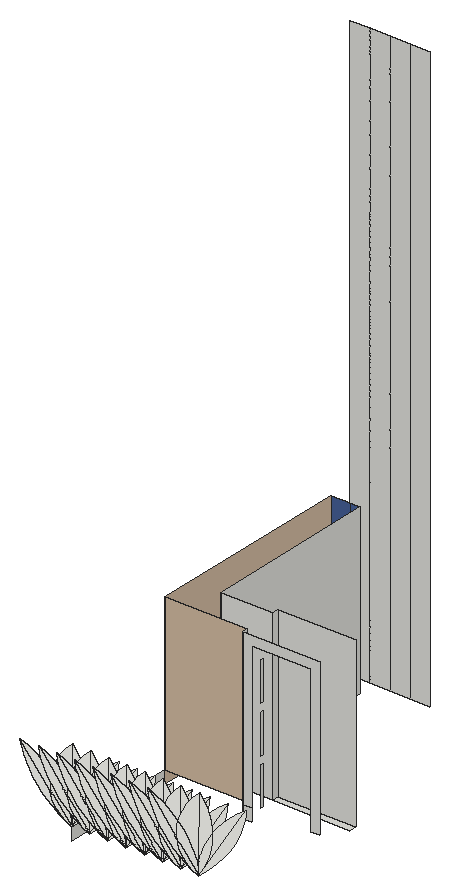
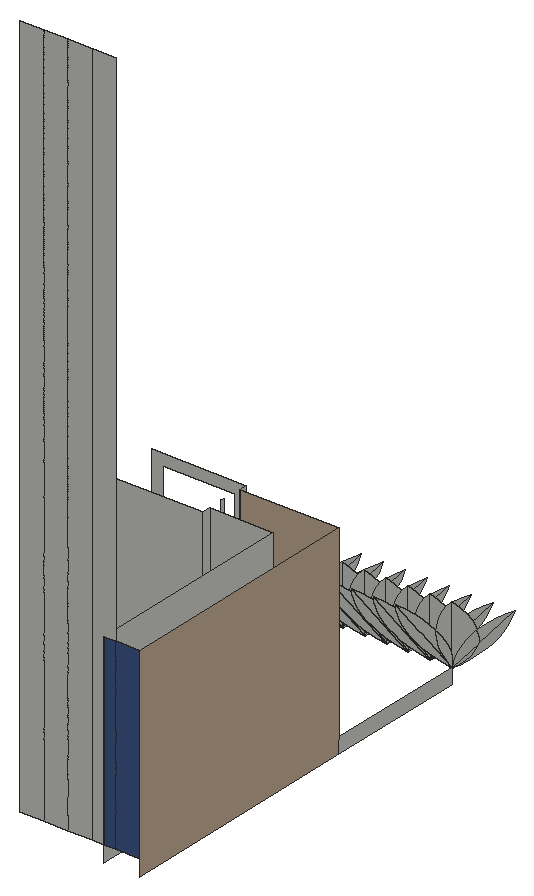
# SketchUp Ruby script. Lengths in inches.
U = 1.inch
M = Sketchup.active_model
def pt(a) = Geom::Point3d.new(a.map { |v| v * U })
def face(e, loops, mat)
  f = e.add_face(loops[0].map { |a| pt(a) })
  loops[1..].each { |l| e.add_face(l.map { |a| pt(a) }).erase! }
  f.material = f.back_material = mat if mat
  f
end
# faces: each face lists its corners as indices into pts; further lists are holes
def faces(e, pts, list, mat = nil) = list.each { |f| face(e, (f[0].is_a?(Array) ? f : [f]).map { |l| l.map { |i| pts[i] } }, mat) }
# xy, xz, yz: faces in a plane at the given z, y or x. An outline is a flat list of corners, or four numbers for a rectangle; further outlines are holes
def ring(l) = l.size == 4 ? [[l[0], l[1]], [l[2], l[1]], [l[2], l[3]], [l[0], l[3]]] : l.each_slice(2).to_a
def flat(e, list, mat, &to3) = list.each { |f| face(e, (f[0].is_a?(Array) ? f : [f]).map { |l| ring(l).map { |u, v| to3.(u, v) } }, mat) }
def xy(e, z, list, mat = nil) = flat(e, list, mat) { |x, y| [x, y, z] }
def xz(e, y, list, mat = nil) = flat(e, list, mat) { |x, z| [x, y, z] }
def yz(e, x, list, mat = nil) = flat(e, list, mat) { |y, z| [x, y, z] }
def lines(e, pts, list) = list.each { |a, b| e.add_line(pt(pts[a]), pt(pts[b])) }
# prism: a flat outline (further loops are holes) pulled along v
def prism(e, loops, v, mat = nil)
  f = face(e, loops, mat); d = Geom::Vector3d.new(v.map { |x| x * U })
  f.pushpull(f.normal.samedirection?(d) ? d.length : -d.length)
end
def box(e, o, s, mat = nil) = prism(e, [[o, [o[0] + s[0], o[1], o[2]], [o[0] + s[0], o[1] + s[1], o[2]], [o[0], o[1] + s[1], o[2]]]], [0, 0, s[2]], mat)
def at(x, y, z, deg = 0) = Geom::Transformation.translation(pt([x, y, z])) * Geom::Transformation.rotation(ORIGIN, Z_AXIS, deg.degrees)
def axes(o, x, y, z) = Geom::Transformation.new([*x, 0, *y, 0, *z, 0, *pt(o).to_a, 1])
def part(name) = M.definitions.add(name)
# library, detail: a bought-in or finely detailed component or shape, given as its bounding box
def library(name, o, s) = part(name).tap { |d| box(d.entities, o, s) }
def detail(e, o, s) = box(e.add_group.entities, o, s)
def put(e, d, t, mat = nil) = e.add_instance(d, t).tap { |i| i.material = mat if mat }
def group(e, t, mat = nil) = e.add_group.tap { |g| g.transformation = t; g.material = mat if mat }.entities
root = M.entities
M.materials.add("[Formica Blue]").color = [71, 97, 152]
M.materials.add("[Formica Laminate Light]").color = [213, 189, 164]
xy(root,-6,[[60.83,69.27,96.11,72.34]])
xz(root,52.17,[[60.83,-6,65.07,-0.3125],[60.83,-0.3125,65.07,-0.3125,65.07,66.01,91.875,66.01,91.875,-0.3125,96.11,-0.3125,96.11,70.25,60.83,70.25]])
xz(root,54.73,[[23.53,-0.3125,60.83,70.25]],"[Formica Laminate Light]")
xz(root,69.27,[[36.96,-6,60.83,70.25]])
xz(root,72.34,[[60.83,-6,96.11,70.25]])
xz(root,148.73,[[36.96,0,41.3,0,41.3,267.125,32.53,267.125,32.53,70.25,36.96,70.25],[41.3,0,50.53,267.125],[50.53,0,59.53,267.125],[59.53,0,68.53,267.125]])
xz(root,148.73,[[23.53,0,32.53,70.25],[32.53,0,36.96,70.25]],"[Formica Blue]")
yz(root,23.53,[[1.54,-6,54.73,-0.3125]])
yz(root,23.53,[[54.73,-6,148.73,70.25]],"[Formica Laminate Light]")
yz(root,36.96,[[69.27,-6,148.73,70.25]])
yz(root,60.83,[[52.17,-6,54.73,-0.3125],[69.27,-6,72.34,70.25],[52.17,-0.3125,54.73,70.25]])
yz(root,70.01,[[51.17,2,52.17,19.625],[51.17,23.34,52.17,40.97],[51.17,44.6875,52.17,62.3125]])
p = [[58.1,2.21,24.34],[56.99,2.71,26.88],[70.57,2.65,10.87],[70.7,2.54,10.46],[71.91,2.12,7.97],[73.51,1.91,5.5625],
  [75.51,1.92,3.27],[77.85,2.15,1.11],[80.53,2.6,-0.87],[77.79,2.13,1.125],[75.17,1.74,3.19],[72.6875,1.4375,5.33],
  [70.34,1.22,7.53],[68.13,1.1,9.79],[66.07,1.0625,12.1],[64.16,1.12,14.47],[62.41,1.26,16.88],[60.81,1.49,19.33],
  [59.37,1.81,21.82],[74.2,10.8125,27.37],[79.4,4.0625,4.15],[79.43,3.87,3.62],[79.84,3.17,1.37],[79.62,3.2,1.71],
  [78.5,3.7,4.27],[77.18,4.08,6.8],[75.66,4.36,9.28],[73.95,4.54,11.72],[72.04,4.6,14.11],[69.96,4.55,16.43],
  [69.6,4.53,16.79],[69.64,5.06,18.08],[70.15,6.27,20.56],[71.09,7.64,22.96],[72.45,9.17,25.23],[69.56,4.02,15.55],
  [69.92,3.18,12.99],[79.3125,4.69,5.86],[79.48,5.65,8.08],[79.9375,6.72,10.27],[80.68,7.9,12.4],[81.48,8.9,14.02],
  [81.65,8.74,13.4],[82.07,7.98,10.98],[82.25,7.11,8.56],[82.18,6.13,6.15],[81.87,5.05,3.77],[81.32,3.87,1.43],
  [88.37,15.11,21.72],[90.63,16.73,23.22],[81.7,9.18,14.46],[82.99,10.55,16.44],[84.54,12,18.32],[86.34,13.52,20.08],
  [90.9375,16.01,21.01],[91.03,15.18,18.81],[90.91,14.27,16.62],[90.57,13.26,14.46],[90.02,12.17,12.33],[89.26,11,10.25],
  [88.3,9.76,8.22],[87.13,8.44,6.25],[85.76,7.0625,4.34],[84.2,5.625,2.52],[82.45,4.14,0.78],[49.96,2.0625,24.42],
  [48.85,2.55,26.96],[62.43,2.5,10.95],[62.56,2.39,10.54],[63.76,1.97,8.05],[65.37,1.76,5.64],[67.36,1.77,3.35],
  [69.71,2,1.19],[72.39,2.45,-0.79],[69.64,1.98,1.21],[67.03,1.59,3.27],[64.54,1.29,5.41],[62.2,1.07,7.61],
  [59.99,0.95,9.87],[57.93,0.91,12.18],[56.02,0.96,14.55],[54.26,1.11,16.96],[52.67,1.34,19.41],[51.23,1.66,21.9],
  [61.42,3.87,15.625],[61.46,4.38,16.87],[61.8125,4.4,16.51],[63.9,4.45,14.1875],[65.81,4.38,11.8],[67.52,4.21,9.36],
  [69.04,3.93,6.875],[70.36,3.54,4.35],[71.48,3.05,1.79],[61.77,3.03,13.07],[66.06,10.66,27.45],[71.26,3.91,4.23],
  [71.29,3.71,3.7],[71.69,3.02,1.45],[61.5,4.9,18.16],[62.01,6.12,20.64],[62.95,7.49,23.03],[64.31,9.01,25.3125],
  [71.17,4.54,5.94],[71.34,5.5,8.16],[71.8,6.57,10.35],[72.54,7.75,12.48],[73.34,8.75,14.1],[73.51,8.58,13.48],
  [73.93,7.83,11.06],[74.11,6.95,8.64],[74.04,5.98,6.23],[73.73,4.9,3.85],[73.18,3.72,1.51],[80.23,14.95,21.8],
  [82.49,16.58,23.29],[73.56,9.03,14.54],[74.84,10.4,16.52],[76.39,11.85,18.4],[78.19,13.37,20.16],[82.79,15.85,21.09],
  [82.89,15.03,18.89],[82.77,14.11,16.7],[82.43,13.11,14.54],[81.88,12.02,12.41],[81.12,10.85,10.33],[80.16,9.6,8.3],
  [78.99,8.29,6.33],[77.62,6.91,4.42],[76.06,5.47,2.6],[74.31,3.99,0.86],[41.82,1.91,24.5],[40.71,2.4,27.04],
  [54.29,2.34,11.03],[54.42,2.24,10.62],[55.62,1.8125,8.13],[57.23,1.61,5.72],[59.22,1.62,3.42],[61.57,1.85,1.27],
  [64.24,2.3,-0.71],[61.5,1.82,1.28],[58.89,1.44,3.35],[56.4,1.13,5.49],[54.05,0.92,7.6875],[51.85,0.8,9.95],
  [49.79,0.76,12.26],[47.88,0.8125,14.63],[46.12,0.95,17.04],[44.52,1.18,19.49],[43.09,1.5,21.98],[57.91,10.51,27.53],
  [63.12,3.76,4.31],[63.15,3.5625,3.78],[63.55,2.86,1.53],[63.34,2.9,1.87],[62.22,3.39,4.43],[60.9,3.78,6.96],
  [59.38,4.0625,9.44],[57.67,4.23,11.88],[55.76,4.3,14.27],[53.67,4.25,16.59],[53.32,4.23,16.95],[53.36,4.75,18.24],
  [53.87,5.97,20.72],[54.81,7.34,23.11],[56.16,8.86,25.39],[53.28,3.72,15.7],[53.63,2.88,13.15],[63.03,4.39,6.02],
  [63.2,5.34,8.24],[63.65,6.42,10.43],[64.4,7.59,12.56],[65.19,8.6,14.18],[65.36,8.43,13.56],[65.79,7.67,11.13],
  [65.96,6.8,8.72],[65.9,5.83,6.3125],[65.59,4.75,3.93],[65.04,3.57,1.59],[72.09,14.8,21.875],[74.34,16.43,23.375],
  [65.41,8.875,14.62],[66.7,10.25,16.6],[68.25,11.7,18.48],[70.05,13.22,20.24],[74.65,15.7,21.17],[74.75,14.88,18.97],
  [74.625,13.96,16.78],[74.29,12.96,14.62],[73.74,11.87,12.49],[72.98,10.7,10.41],[72.01,9.45,8.375],[70.84,8.14,6.41],
  [69.47,6.76,4.5],[67.91,5.32,2.68],[66.17,3.83,0.9375],[25.53,1.61,24.66],[24.43,2.1,27.2],[38.01,2.04,11.1875],
  [38.13,1.9375,10.77],[39.34,1.51,8.29],[40.95,1.3,5.88],[42.9375,1.31,3.58],[45.29,1.55,1.43],[47.96,2,-0.55],
  [45.22,1.52,1.44],[42.6,1.13,3.51],[40.12,0.83,5.65],[37.77,0.62,7.85],[35.5625,0.49,10.11],[33.5,0.46,12.42],
  [31.59,0.51,14.79],[29.84,0.65,17.2],[28.24,0.88,19.65],[26.8,1.2,22.14],[33.67,1.76,24.58],[32.57,2.25,27.12],
  [46.15,2.19,11.11],[46.27,2.09,10.7],[47.48,1.66,8.21],[49.09,1.45,5.8],[51.08,1.47,3.5],[53.43,1.7,1.35],
  [56.1,2.15,-0.63],[53.36,1.67,1.36],[50.74,1.28,3.43],[48.26,0.98,5.57],[45.91,0.77,7.77],[43.71,0.64,10.03],
  [41.65,0.61,12.34],[39.74,0.66,14.71],[37.98,0.8,17.12],[36.38,1.03,19.57],[34.95,1.35,22.06],[41.63,10.2,27.68],
  [46.83,3.46,4.47],[46.86,3.26,3.93],[47.27,2.56,1.6875],[47.05,2.6,2.03],[45.9375,3.09,4.59],[44.62,3.48,7.11],
  [43.1,3.76,9.6],[41.38,3.93,12.04],[39.48,3.99,14.43],[37.39,3.95,16.75],[37.03,3.92,17.1],[37.07,4.45,18.4],
  [37.59,5.66,20.875],[38.53,7.04,23.27],[39.88,8.56,25.55],[36.99,3.42,15.86],[37.35,2.57,13.3125],[46.74,4.09,6.18],
  [46.91,5.04,8.4],[47.37,6.11,10.59],[48.11,7.29,12.72],[48.91,8.3,14.34],[49.08,8.13,13.71],[49.5,7.37,11.29],
  [49.68,6.5,8.875],[49.61,5.52,6.47],[49.3,4.44,4.09],[48.75,3.27,1.75],[55.8,14.5,22.04],[58.0625,16.125,23.53],
  [49.13,8.57,14.78],[50.42,9.94,16.76],[51.97,11.4,18.64],[53.77,12.92,20.4],[58.37,15.4,21.33],[58.46,14.57,19.125],
  [58.34,13.66,16.94],[58.01,12.65,14.78],[57.46,11.5625,12.65],[56.7,10.39,10.57],[55.73,9.15,8.54],[54.56,7.83,6.5625],
  [53.19,6.46,4.66],[51.63,5.02,2.84],[49.88,3.53,1.1],[45.13,3.57,15.78],[45.17,4.07,17.03],[45.53,4.1,16.67],
  [47.62,4.14,14.35],[49.52,4.08,11.96],[51.24,3.91,9.52],[52.76,3.63,7.04],[54.08,3.24,4.51],[55.19,2.75,1.95],
  [45.49,2.73,13.23],[49.77,10.36,27.61],[54.98,3.61,4.39],[55,3.41,3.85],[55.41,2.71,1.61],[45.21,4.6,18.32],
  [45.73,5.8125,20.8],[46.67,7.1875,23.19],[48.02,8.71,25.47],[54.89,4.24,6.1],[55.06,5.19,8.32],[55.51,6.26,10.51],
  [56.25,7.44,12.64],[57.05,8.45,14.26],[57.22,8.28,13.64],[57.64,7.52,11.21],[57.82,6.65,8.8],[57.76,5.67,6.39],
  [57.45,4.59,4.01],[56.89,3.42,1.67],[63.95,14.65,21.96],[66.2,16.28,23.45],[57.27,8.72,14.7],[58.5625,10.09,16.68],
  [60.11,11.55,18.56],[61.91,13.07,20.32],[66.51,15.55,21.25],[66.6,14.73,19.05],[66.48,13.81,16.86],[66.15,12.8,14.7],
  [65.6,11.71,12.57],[64.84,10.54,10.49],[63.87,9.3,8.46],[62.7,7.99,6.48],[61.33,6.61,4.58],[59.77,5.17,2.76],
  [58.03,3.68,1.02],[17.39,1.45,24.73],[16.28,1.95,27.28],[29.86,1.89,11.27],[29.99,1.78,10.85],[31.2,1.36,8.37],
  [32.8,1.15,5.96],[34.8,1.16,3.66],[37.14,1.4,1.51],[39.82,1.85,-0.47],[37.08,1.37,1.52],[34.46,0.98,3.59],
  [31.98,0.68,5.72],[29.63,0.46,7.92],[27.42,0.34,10.18],[25.36,0.3,12.5],[23.45,0.36,14.87],[21.7,0.5,17.28],
  [20.1,0.73,19.73],[18.66,1.05,22.22],[33.49,10.05,27.76],[38.69,3.3,4.55],[38.72,3.11,4.01],[39.125,2.41,1.76],
  [38.91,2.44,2.11],[37.79,2.9375,4.67],[36.47,3.33,7.19],[34.95,3.61,9.68],[33.24,3.78,12.12],[31.33,3.84,14.51],
  [29.25,3.79,16.83],[28.89,3.77,17.18],[28.93,4.3,18.48],[29.44,5.51,20.96],[30.38,6.89,23.35],[31.74,8.41,25.63],
  [28.85,3.26,15.94],[29.21,2.42,13.39],[38.6,3.94,6.26],[38.77,4.89,8.48],[39.23,5.96,10.67],[39.97,7.14,12.8],
  [40.77,8.14,14.42],[40.9375,7.98,13.79],[41.36,7.22,11.37],[41.54,6.35,8.95],[41.47,5.37,6.55],[41.16,4.29,4.17],
  [40.61,3.11,1.83],[47.66,14.35,22.11],[49.92,15.97,23.61],[40.99,8.42,14.86],[42.28,9.79,16.84],[43.83,11.24,18.71],
  [45.625,12.77,20.48],[50.23,15.25,21.41],[50.32,14.42,19.2],[50.2,13.51,17.02],[49.86,12.5,14.86],[49.3125,11.41,12.73],
  [48.55,10.24,10.65],[47.59,9,8.61],[46.42,7.68,6.64],[45.05,6.3,4.74],[43.49,4.87,2.92],[41.74,3.38,1.18],
  [9.25,1.3,24.8125],[8.14,1.79,27.36],[21.72,1.74,11.34],[21.85,1.63,10.93],[23.05,1.21,8.44],[24.66,1,6.04],
  [26.65,1.01,3.74],[29,1.24,1.59],[31.68,1.69,-0.39],[28.93,1.22,1.6],[26.32,0.83,3.67],[23.83,0.53,5.8],
  [21.49,0.3125,8],[19.28,0.1875,10.26],[17.22,0.15,12.58],[15.31,0.2,14.95],[13.55,0.35,17.36],[11.96,0.58,19.81],
  [10.52,0.9,22.3],[25.35,9.9,27.84],[30.55,3.15,4.625],[30.58,2.95,4.09],[30.98,2.26,1.84],[30.77,2.29,2.1875],
  [29.65,2.79,4.75],[28.33,3.17,7.27],[26.8125,3.45,9.76],[25.1,3.625,12.2],[23.19,3.6875,14.58],[21.1,3.64,16.91],
  [20.75,3.62,17.26],[20.79,4.15,18.55],[21.3,5.36,21.03],[22.24,6.73,23.43],[23.6,8.25,25.71],[20.71,3.11,16.02],
  [21.0625,2.27,13.47],[30.46,3.78,6.34],[30.63,4.74,8.56],[31.09,5.81,10.75],[31.83,6.99,12.88],[32.625,7.99,14.49],
  [32.8,7.83,13.87],[33.22,7.07,11.45],[33.4,6.2,9.03],[33.33,5.22,6.63],[33.02,4.14,4.25],[32.47,2.96,1.91],
  [39.52,14.19,22.19],[41.78,15.82,23.69],[32.85,8.27,14.9375],[34.14,9.64,16.92],[35.69,11.09,18.79],[37.48,12.61,20.56],
  [42.08,15.09,21.48],[42.18,14.27,19.28],[42.06,13.35,17.1],[41.72,12.35,14.9375],[41.17,11.26,12.81],[40.41,10.09,10.73],
  [39.45,8.84,8.69],[38.28,7.53,6.72],[36.91,6.15,4.82],[35.35,4.72,2.99],[33.6,3.23,1.26],[1.11,1.15,24.89],
  [0,1.64,27.4375],[13.58,1.58,11.42],[13.71,1.48,11.01],[14.91,1.06,8.52],[16.52,0.85,6.12],[18.51,0.86,3.82],
  [20.86,1.09,1.67],[23.53,1.54,-0.3125],[20.79,1.07,1.68],[18.18,0.68,3.75],[15.69,0.375,5.88],[13.34,0.16,8.08],
  [11.14,0.04,10.34],[9.08,0,12.66],[7.17,0.05,15.02],[5.41,0.19,17.4375],[3.81,0.43,19.89],[2.38,0.74,22.375],
  [12.57,2.96,16.1],[12.61,3.47,17.34],[12.96,3.49,16.99],[15.05,3.54,14.66],[16.96,3.47,12.28],[18.67,3.3,9.84],
  [20.19,3.02,7.35],[21.51,2.63,4.83],[22.625,2.14,2.27],[12.92,2.12,13.55],[17.21,9.75,27.92],[22.41,3,4.71],
  [22.4375,2.8,4.17],[22.84,2.1,1.92],[12.65,3.99,18.63],[13.16,5.21,21.11],[14.1,6.58,23.51],[15.45,8.1,25.79],
  [22.32,3.63,6.42],[22.49,4.59,8.64],[22.94,5.66,10.82],[23.69,6.84,12.96],[24.48,7.84,14.57],[24.65,7.67,13.95],
  [25.08,6.91,11.53],[25.25,6.04,9.11],[25.1875,5.07,6.71],[24.88,3.99,4.33],[24.33,2.81,1.98],[31.38,14.04,22.27],
  [33.63,15.67,23.77],[24.7,8.12,15.02],[25.99,9.49,17],[27.54,10.94,18.87],[29.34,12.46,20.64],[33.94,14.94,21.5625],
  [34.04,14.12,19.36],[33.92,13.2,17.18],[33.58,12.2,15.02],[33.03,11.11,12.89],[32.27,9.9375,10.8],[31.3,8.69,8.77],
  [30.13,7.38,6.8],[28.77,6,4.9],[27.2,4.5625,3.07],[25.46,3.08,1.33],[72.84,9.23,15.89],[67.86,10.62,25.24],
  [69.44,10.45,22.97],[70.81,10.17,20.65],[71.94,9.76,18.28],[80.99,9.38,15.8125],[76,10.77,25.16],[77.59,10.61,22.89],
  [78.95,10.32,20.57],[80.09,9.91,18.2],[64.7,9.08,15.97],[59.72,10.47,25.32],[61.3,10.3,23.05],[62.67,10.02,20.73],
  [63.8,9.61,18.36],[56.56,8.93,16.05],[51.57,10.31,25.4],[53.16,10.15,23.13],[54.52,9.86,20.81],[55.66,9.45,18.44],
  [40.28,8.62,16.21],[35.29,10.01,25.56],[36.88,9.85,23.29],[38.24,9.56,20.96],[39.375,9.15,18.6],[48.42,8.77,16.13],
  [43.43,10.16,25.48],[45.02,10,23.21],[46.38,9.71,20.88],[47.52,9.3,18.52],[32.13,8.47,16.29],[27.15,9.86,25.64],
  [28.74,9.69,23.37],[30.1,9.41,21.04],[31.23,9,18.68],[23.99,8.32,16.37],[19.01,9.71,25.71],[20.59,9.54,23.44],
  [21.96,9.26,21.12],[23.09,8.85,18.76],[51.75,3.14,25.05],[54.51,3.61,23.04],[57.11,3.98,20.95],[59.55,4.25,18.77],
  [59.9,3.29,24.97],[62.65,3.76,22.96],[65.25,4.14,20.87],[67.6875,4.4,18.6875],[43.61,2.98,25.13],[46.37,3.46,23.12],
  [48.97,3.83,21.02],[51.41,4.1,18.85],[35.47,2.83,25.21],[38.23,3.31,23.2],[40.83,3.68,21.1],[43.26,3.94,18.93],
  [27.33,2.68,25.29],[30.08,3.16,23.28],[32.68,3.53,21.18],[35.12,3.79,19],[11.04,2.375,25.44],[13.8,2.85,23.4375],
  [16.4,3.22,21.34],[18.84,3.49,19.16],[19.1875,2.53,25.37],[21.94,3.01,23.36],[24.54,3.375,21.26],[26.98,3.64,19.08],
  [2.9,2.22,25.52],[5.66,2.7,23.52],[8.26,3.07,21.42],[10.7,3.34,19.24]]
faces(root,p,[[0,1,2,3,4,5,6,7,8,9,10,11,12,13,14,15,16,17,18],[3,2,8,7,6,5,4],[19,20,21,22,8,23,24,25,26,27,28,29,30,31,32,33,34],[35,30,29,28,27,26,25,24,23,8,2,36],[8,20,37,38,39,40,41,42,43,44,45,46,47],[20,8,22,21],[48,49,8,47,46,45,44,43,42,41,50,51,52,53],[8,49,54,55,56,57,58,59,60,61,62,63,64],
  [65,66,67,68,69,70,71,72,73,74,75,76,77,78,79,80,81,82,83],[68,67,73,72,71,70,69],[84,85,86,87,88,89,90,91,92,73,67,93],[94,95,96,97,73,92,91,90,89,88,87,86,85,98,99,100,101],[73,95,102,103,104,105,106,107,108,109,110,111,112],[95,73,97,96],[113,114,73,112,111,110,109,108,107,106,115,116,117,118],[73,114,119,120,121,122,123,124,125,126,127,128,129],
  [130,131,132,133,134,135,136,137,138,139,140,141,142,143,144,145,146,147,148],[133,132,138,137,136,135,134],[149,150,151,152,138,153,154,155,156,157,158,159,160,161,162,163,164],[165,160,159,158,157,156,155,154,153,138,132,166],[138,150,167,168,169,170,171,172,173,174,175,176,177],[150,138,152,151],[178,179,138,177,176,175,174,173,172,171,180,181,182,183],[138,179,184,185,186,187,188,189,190,191,192,193,194],
  [195,196,197,198,199,200,201,202,203,204,205,206,207,208,209,210,211,212,213],[214,215,216,217,218,219,220,221,222,223,224,225,226,227,228,229,230,231,232],[198,197,203,202,201,200,199],[217,216,222,221,220,219,218],[233,234,235,236,203,237,238,239,240,241,242,243,244,245,246,247,248],[249,244,243,242,241,240,239,238,237,203,197,250],[203,234,251,252,253,254,255,256,257,258,259,260,261],[234,203,236,235],
  [262,263,203,261,260,259,258,257,256,255,264,265,266,267],[203,263,268,269,270,271,272,273,274,275,276,277,278],[279,280,281,282,283,284,285,286,287,222,216,288],[289,290,291,292,222,287,286,285,284,283,282,281,280,293,294,295,296],[222,290,297,298,299,300,301,302,303,304,305,306,307],[290,222,292,291],[308,309,222,307,306,305,304,303,302,301,310,311,312,313],[222,309,314,315,316,317,318,319,320,321,322,323,324],
  [325,326,327,328,329,330,331,332,333,334,335,336,337,338,339,340,341,342,343],[328,327,333,332,331,330,329],[344,345,346,347,333,348,349,350,351,352,353,354,355,356,357,358,359],[360,355,354,353,352,351,350,349,348,333,327,361],[333,345,362,363,364,365,366,367,368,369,370,371,372],[345,333,347,346],[373,374,333,372,371,370,369,368,367,366,375,376,377,378],[333,374,379,380,381,382,383,384,385,386,387,388,389],
  [390,391,392,393,394,395,396,397,398,399,400,401,402,403,404,405,406,407,408],[393,392,398,397,396,395,394],[409,410,411,412,398,413,414,415,416,417,418,419,420,421,422,423,424],[425,420,419,418,417,416,415,414,413,398,392,426],[398,410,427,428,429,430,431,432,433,434,435,436,437],[410,398,412,411],[438,439,398,437,436,435,434,433,432,431,440,441,442,443],[398,439,444,445,446,447,448,449,450,451,452,453,454],
  [455,456,457,458,459,460,461,462,463,464,465,466,467,468,469,470,471,472,473],[458,457,463,462,461,460,459],[474,475,476,477,478,479,480,481,482,463,457,483],[484,485,486,487,463,482,481,480,479,478,477,476,475,488,489,490,491],[463,485,492,493,494,495,496,497,498,499,500,501,502],[485,463,487,486],[503,504,463,502,501,500,499,498,497,496,505,506,507,508],[463,504,509,510,511,512,513,514,515,516,517,518,519],
  [520,106,105,104,103,102,95,94,521,522,523,524],[525,41,40,39,38,37,20,19,526,527,528,529],[530,171,170,169,168,167,150,149,531,532,533,534],[535,301,300,299,298,297,290,289,536,537,538,539],[540,366,365,364,363,362,345,344,541,542,543,544],[545,255,254,253,252,251,234,233,546,547,548,549],[550,431,430,429,428,427,410,409,551,552,553,554],[555,496,495,494,493,492,485,484,556,557,558,559],
  [67,66,560,561,562,563,85,84,93],[2,1,564,565,566,567,30,35,36],[132,131,568,569,570,571,160,165,166],[216,215,572,573,574,575,280,279,288],[197,196,576,577,578,579,244,249,250],[392,391,580,581,582,583,420,425,426],[327,326,584,585,586,587,355,360,361],[457,456,588,589,590,591,475,474,483]])
